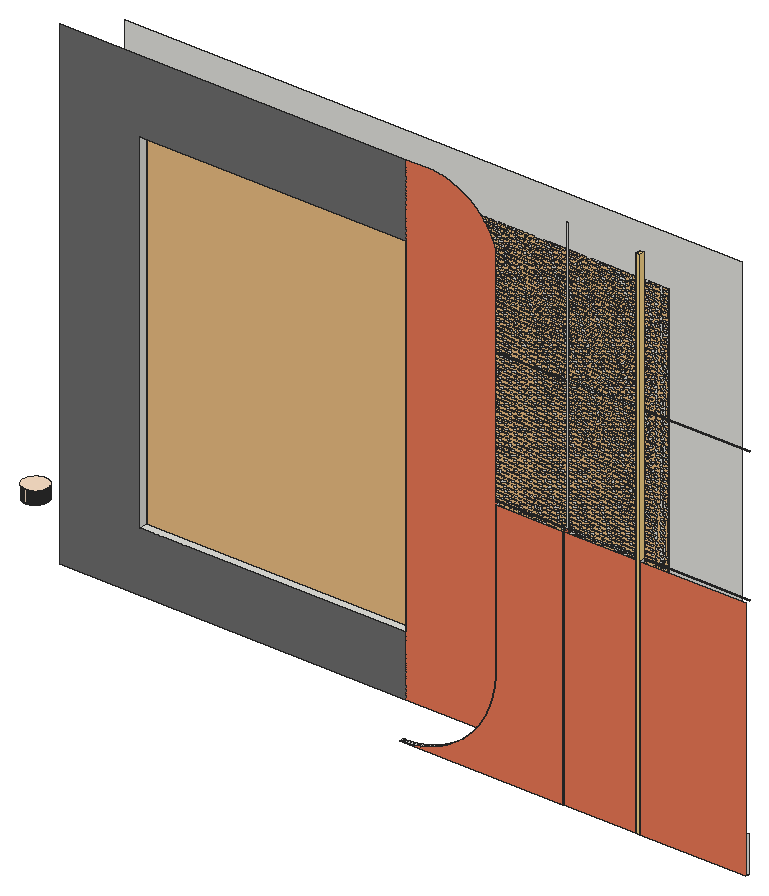
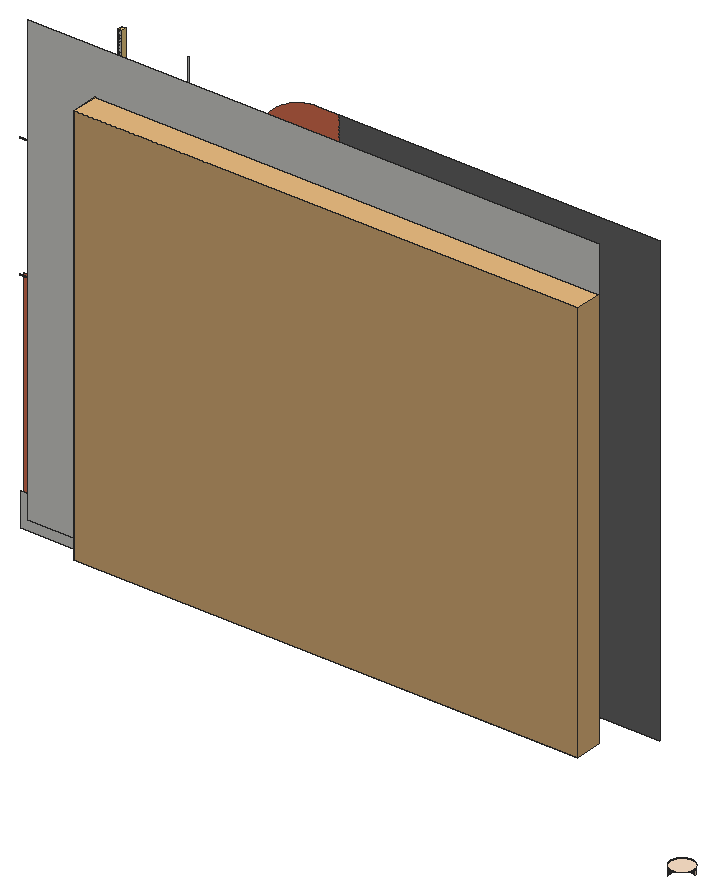
# SketchUp Ruby script. Lengths in inches.
U = 1.inch
M = Sketchup.active_model
def pt(a) = Geom::Point3d.new(a.map { |v| v * U })
def face(e, loops, mat)
  f = e.add_face(loops[0].map { |a| pt(a) })
  loops[1..].each { |l| e.add_face(l.map { |a| pt(a) }).erase! }
  f.material = f.back_material = mat if mat
  f
end
# faces: each face lists its corners as indices into pts; further lists are holes
def faces(e, pts, list, mat = nil) = list.each { |f| face(e, (f[0].is_a?(Array) ? f : [f]).map { |l| l.map { |i| pts[i] } }, mat) }
# xy, xz, yz: faces in a plane at the given z, y or x. An outline is a flat list of corners, or four numbers for a rectangle; further outlines are holes
def ring(l) = l.size == 4 ? [[l[0], l[1]], [l[2], l[1]], [l[2], l[3]], [l[0], l[3]]] : l.each_slice(2).to_a
def flat(e, list, mat, &to3) = list.each { |f| face(e, (f[0].is_a?(Array) ? f : [f]).map { |l| ring(l).map { |u, v| to3.(u, v) } }, mat) }
def xy(e, z, list, mat = nil) = flat(e, list, mat) { |x, y| [x, y, z] }
def xz(e, y, list, mat = nil) = flat(e, list, mat) { |x, z| [x, y, z] }
def yz(e, x, list, mat = nil) = flat(e, list, mat) { |y, z| [x, y, z] }
def lines(e, pts, list) = list.each { |a, b| e.add_line(pt(pts[a]), pt(pts[b])) }
# prism: a flat outline (further loops are holes) pulled along v
def prism(e, loops, v, mat = nil)
  f = face(e, loops, mat); d = Geom::Vector3d.new(v.map { |x| x * U })
  f.pushpull(f.normal.samedirection?(d) ? d.length : -d.length)
end
def box(e, o, s, mat = nil) = prism(e, [[o, [o[0] + s[0], o[1], o[2]], [o[0] + s[0], o[1] + s[1], o[2]], [o[0], o[1] + s[1], o[2]]]], [0, 0, s[2]], mat)
def at(x, y, z, deg = 0) = Geom::Transformation.translation(pt([x, y, z])) * Geom::Transformation.rotation(ORIGIN, Z_AXIS, deg.degrees)
def axes(o, x, y, z) = Geom::Transformation.new([*x, 0, *y, 0, *z, 0, *pt(o).to_a, 1])
def part(name) = M.definitions.add(name)
# library, detail: a bought-in or finely detailed component or shape, given as its bounding box
def library(name, o, s) = part(name).tap { |d| box(d.entities, o, s) }
def detail(e, o, s) = box(e.add_group.entities, o, s)
def put(e, d, t, mat = nil) = e.add_instance(d, t).tap { |i| i.material = mat if mat }
def group(e, t, mat = nil) = e.add_group.tap { |g| g.transformation = t; g.material = mat if mat }.entities
root = M.entities
M.materials.add("1122 AP 7994 PEACH ROSE").color = [254, 227, 201]
M.materials.add("Wall Light").color = [248, 213, 137]
M.materials.add("[Formica Beige]").color = [235, 120, 86]
M.materials.add("[Stone Flagstone Ashlar]").color = [109, 109, 109]
c1 = library("Component",[73.72,0,0],[62.99,4.72,84.625])
c2 = library("Component_63",[0,-41.05,1.35],[7.23,156.73,136.43])
xy(root,149.82,[[280.17,152,280.52,153],[280.17,152,320.75,153],[321,152,338.75,153],[339.75,152,366,153]])
xy(root,152.82,[[164.79,180.07,164.72,180.08,164.4,180.12,164.33,180.14,164.25,180.15,164.17,180.17,164.1,180.19,164.02,180.22,163.95,180.24,163.8,180.3,163.66,180.36,163.59,180.4,163.52,180.43,163.38,180.51,163.32,180.55,163.25,180.6,163.1875,180.64,163,180.79,162.94,180.84,162.83,180.95,162.78,181.01,162.72,181.0625,162.67,181.12,162.57,181.24,162.52,181.31,162.48,181.37,162.44,181.4375,162.39,181.5,162.31,181.64,162.28,181.71,162.24,181.78,162.18,181.92,162.15,182,162.1,182.14,162.07,182.22,162.05,182.29,162.03,182.37,162.02,182.45,162,182.52,161.96,182.84,161.96,182.91,161.95,182.99,161.95,183.15,161.96,183.23,161.96,183.31,161.97,183.38,162,183.62,162.02,183.69,162.03,183.77,162.05,183.85,162.07,183.92,162.1,184,162.125,184.07,162.15,184.15,162.24,184.36,162.28,184.43,162.31,184.5,162.39,184.64,162.44,184.7,162.48,184.77,162.52,184.83,162.57,184.9,162.72,185.08,162.94,185.3,163,185.35,163.1875,185.5,163.25,185.54,163.32,185.59,163.38,185.63,163.52,185.71,163.59,185.74,163.66,185.78,163.73,185.8125,163.8,185.84,163.95,185.9,164.02,185.92,164.1,185.95,164.17,185.97,164.33,186.01,164.4,186.02,164.48,186.03,164.56,186.05,164.64,186.05,164.72,186.0625,164.79,186.07,165.11,186.07,165.1875,186.0625,165.26,186.05,165.34,186.05,165.42,186.03,165.5,186.02,165.57,186.01,165.73,185.97,165.8,185.95,165.88,185.92,165.95,185.9,166.03,185.87,166.1,185.84,166.17,185.8125,166.24,185.78,166.3125,185.74,166.38,185.71,166.59,185.59,166.65,185.54,166.71,185.5,166.78,185.45,167.02,185.25,167.07,185.19,167.13,185.14,167.33,184.9,167.38,184.83,167.42,184.77,167.47,184.7,167.51,184.64,167.59,184.5,167.66,184.36,167.75,184.15,167.78,184.07,167.8,184,167.83,183.92,167.85,183.85,167.89,183.69,167.9,183.62,167.91,183.54,167.93,183.46,167.93,183.38,167.94,183.31,167.95,183.23,167.95,182.91,167.94,182.84,167.93,182.76,167.93,182.68,167.91,182.6,167.9,182.52,167.89,182.45,167.85,182.29,167.83,182.22,167.8,182.14,167.78,182.07,167.75,182,167.72,181.92,167.66,181.78,167.59,181.64,167.51,181.5,167.47,181.4375,167.42,181.37,167.38,181.31,167.33,181.24,167.23,181.12,167.18,181.0625,167.13,181.01,167.07,180.95,167.02,180.89,166.78,180.69,166.71,180.64,166.65,180.6,166.59,180.55,166.38,180.43,166.3125,180.4,166.24,180.36,166.03,180.27,165.95,180.24,165.88,180.22,165.8,180.19,165.73,180.17,165.65,180.15,165.57,180.14,165.5,180.12,165.26,180.09,165.1875,180.08,165.11,180.07]],"1122 AP 7994 PEACH ROSE")
xy(root,173.82,[[215,153,281,162]])
xz(root,152,[[280.17,149.82,320.75,149.82,320.75,210.57,304,210.57,304,173.17,303.99,172.85,303.97,172.52,303.96,172.2,303.93,171.875,303.91,171.55,303.88,171.23,303.76,170.27,303.71,169.95,303.66,169.625,303.6,169.31,303.54,168.99,303.47,168.67,303.4,168.36,303.33,168.04,303.25,167.73,303.17,167.41,302.9,166.48,302.8,166.17,302.69,165.86,302.47,165.26,302.36,164.95,302.24,164.65,302.11,164.35,301.98,164.06,301.85,163.76,301.71,163.47,301.57,163.17,301.43,162.88,301.28,162.6,301.13,162.31,300.97,162.03,300.8125,161.74,300.65,161.46,300.48,161.1875,300.31,160.91,300.13,160.64,299.96,160.37,299.77,160.1,299.59,159.84,299.4,159.57,299.2,159.3125,299.01,159.06,298.79,158.82,298.58,158.52,298.36,158.25,298.12,157.98,297.89,157.71,297.65,157.45,297.4,157.1875,297.15,156.93,296.9,156.68,296.64,156.43,296.39,156.1875,296.12,155.95,295.86,155.71,295.58,155.48,295.3125,155.25,295.03,155.02,294.75,154.8,294.47,154.59,294.18,154.375,293.89,154.17,293.6,153.96,293.3,153.77,293,153.57,292.7,153.38,292.4,153.2,291.78,152.84,291.47,152.67,291.15,152.5,290.51,152.18,289.87,151.88,289.21,151.6,288.55,151.34,288.21,151.22,287.875,151.1,287.54,150.99,287.2,150.88,286.85,150.78,286.51,150.68,286.17,150.59,285.82,150.5,285.47,150.42,285.125,150.34,284.78,150.27,284.43,150.2,284.07,150.14,283.37,150.04,283.01,149.99,282.66,149.95,282.31,149.92,281.59,149.86,281.24,149.84,280.52,149.82],[321,149.82,338.75,210.57],[339.75,149.82,366,210.57]],"[Formica Beige]")
xz(root,153,[[280.17,149.82,280.52,149.82,280.88,149.83,281,149.83,281,149.82],[281,149.82,281,149.83,281.24,149.84,281.59,149.86,282.31,149.92,282.66,149.95,283.01,149.99,283.37,150.04,284.07,150.14,284.43,150.2,284.78,150.27,285.125,150.34,285.47,150.42,285.82,150.5,286.17,150.59,286.51,150.68,286.85,150.78,287.2,150.88,287.54,150.99,287.875,151.1,288.21,151.22,288.55,151.34,289.21,151.6,289.87,151.88,290.51,152.18,291.15,152.5,291.47,152.67,291.78,152.84,292.4,153.2,292.7,153.38,293,153.57,293.3,153.77,293.6,153.96,293.89,154.17,294.18,154.375,294.47,154.59,294.75,154.8,295.03,155.02,295.3125,155.25,295.58,155.48,295.86,155.71,296.12,155.95,296.39,156.1875,296.64,156.43,296.9,156.68,297.15,156.93,297.4,157.1875,297.65,157.45,297.89,157.71,298.12,157.98,298.36,158.25,298.58,158.52,298.79,158.82,320.75,158.82,320.75,149.82],[321,149.82,338.75,158.82],[339.75,149.82,366,158.82]])
xz(root,153,[[281,158.82,298.79,158.82,299.01,159.06,299.2,159.3125,299.4,159.57,299.59,159.84,299.77,160.1,299.96,160.37,300.13,160.64,300.31,160.91,300.48,161.1875,300.65,161.46,300.8125,161.74,300.97,162.03,301.13,162.31,301.28,162.6,301.43,162.88,301.57,163.17,301.71,163.47,301.85,163.76,301.98,164.06,302.11,164.35,302.24,164.65,302.36,164.95,302.47,165.26,302.69,165.86,302.8,166.17,302.9,166.48,303.17,167.41,303.25,167.73,303.33,168.04,303.4,168.36,303.47,168.67,303.54,168.99,303.6,169.31,303.66,169.625,303.71,169.95,303.76,170.27,303.88,171.23,303.91,171.55,303.93,171.875,303.96,172.2,303.97,172.52,303.99,172.85,304,173.17,304,210.57,303,210.57,303,266.72,302.94,267,302.85,267.26,302.75,267.52,302.64,267.77,302.54,268.03,302.42,268.28,302.31,268.54,302.1875,268.79,302.07,269.03,301.9375,269.28,301.81,269.52,301.67,269.77,301.53,270.01,301.39,270.24,301.24,270.48,301.1,270.71,300.94,270.94,300.79,271.17,300.625,271.4,300.46,271.62,300.29,271.84,300.12,272.0625,299.95,272.28,299.41,272.91,299.22,273.11,299.03,273.3125,298.84,273.51,298.64,273.71,298.24,274.09,298.03,274.28,297.4,274.82,296.74,275.33,296.52,275.49,296.29,275.65,296.0625,275.8,295.83,275.96,295.6,276.1,295.36,276.25,294.88,276.53,294.64,276.66,294.39,276.79,294.15,276.92,293.65,277.16,293.39,277.27,293.14,277.39,292.88,277.49,292.625,277.6,292.37,277.69,292.11,277.79,291.85,277.88,291.58,277.97,291.32,278.05,291.05,278.13,290.78,278.2,290.52,278.27,290.25,278.34,289.71,278.46,289.43,278.51,289.16,278.56,288.89,278.6,288.61,278.65,288.34,278.68,288.0625,278.71,287.79,278.74,287.51,278.77,287.23,278.78,286.96,278.8,286.68,278.8125,286.4,278.82,281,278.82]],"[Formica Beige]")
xz(root,153,[[195,158.82,281,158.82,281,173.82,215,173.82,215,260.82,281,260.82,281,278.82,195,278.82]],"[Stone Flagstone Ashlar]")
xz(root,153.25,[[[320.75,158.82,321,158.82,321,210.57,338.75,210.57,338.75,158.82,339.75,158.82,339.75,210.57,366,210.57,366,210.82,339.75,210.82,339.75,243.57,366,243.57,366,243.82,339.75,243.82,339.75,278.82,338.75,278.82,338.75,243.82,321,243.82,321,278.82,320.75,278.82,320.75,243.82,303,243.82,303,243.57,320.75,243.57,320.75,210.82,303,210.82,303,210.57,320.75,210.57],[321,210.82,338.75,243.57]]])
xz(root,162,[[[204,158.82,357,278.82],[215,173.82,281,260.82]]])
xz(root,180.07,[[164.79,149.82,164.87,152.82],[164.87,149.82,164.95,152.82],[164.95,149.82,165.03,152.82],[165.03,149.82,165.11,152.82]],"1122 AP 7994 PEACH ROSE")
yz(root,167.93,[[182.68,149.82,182.76,152.82],[183.38,149.82,183.46,152.82]],"1122 AP 7994 PEACH ROSE")
yz(root,167.95,[[182.91,149.82,182.99,152.82],[182.99,149.82,183.07,152.82],[183.07,149.82,183.15,152.82],[183.15,149.82,183.23,152.82]],"1122 AP 7994 PEACH ROSE")
yz(root,215,[[153,173.82,162,260.82]])
yz(root,281,[[153,173.82,162,260.82]])
yz(root,304,[[152,173.17,153,173.5],[152,173.5,153,173.65],[152,173.65,153,173.82],[152,173.82,153,210.57]])
yz(root,320.75,[[152,149.82,153,158.82]])
yz(root,320.75,[[152,158.82,153.25,210.57]],"[Formica Beige]")
yz(root,321,[[152,149.82,152,210.57,153.25,210.57,153.25,158.82,153,158.82,153,149.82]],"[Formica Beige]")
yz(root,338.75,[[152,149.82,153,149.82,153,158.82,153.25,158.82,153.25,210.57,152,210.57]])
yz(root,339.75,[[152,149.82,152,210.57,153.25,210.57,153.25,158.82,153,158.82,153,149.82]])
p = [[280.88,153,149.83],[280.52,153,149.82],[280.52,152,149.82],[280.88,152,149.83],[281,153,149.83],[281.24,152,149.84],
  [281.24,153,149.84],[281.59,153,149.86],[281.59,152,149.86],[164.33,180.14,149.82],[164.25,180.15,149.82],[164.25,180.15,152.82],
  [164.33,180.14,152.82],[164.4,180.12,149.82],[164.4,180.12,152.82],[164.48,180.11,149.82],[164.48,180.11,152.82],[164.56,180.1,149.82],
  [164.56,180.1,152.82],[164.64,180.09,149.82],[164.64,180.09,152.82],[164.72,180.08,149.82],[164.72,180.08,152.82],[164.79,180.07,149.82],
  [164.79,180.07,152.82],[165.1875,180.08,149.82],[165.11,180.07,149.82],[165.11,180.07,152.82],[165.1875,180.08,152.82],[165.26,180.09,149.82],
  [165.26,180.09,152.82],[165.34,180.1,149.82],[165.34,180.1,152.82],[165.42,180.11,149.82],[165.42,180.11,152.82],[165.5,180.12,149.82],
  [165.5,180.12,152.82],[165.57,180.14,149.82],[165.57,180.14,152.82],[165.65,180.15,149.82],[165.65,180.15,152.82],[163.95,180.24,149.82],
  [163.875,180.27,149.82],[163.875,180.27,152.82],[163.95,180.24,152.82],[164.02,180.22,149.82],[164.02,180.22,152.82],[164.1,180.19,149.82],
  [164.1,180.19,152.82],[164.17,180.17,149.82],[164.17,180.17,152.82],[165.73,180.17,149.82],[165.73,180.17,152.82],[165.8,180.19,149.82],
  [165.8,180.19,152.82],[165.88,180.22,149.82],[165.88,180.22,152.82],[165.95,180.24,149.82],[165.95,180.24,152.82],[166.03,180.27,149.82],
  [166.03,180.27,152.82],[163.73,180.33,149.82],[163.66,180.36,149.82],[163.66,180.36,152.82],[163.73,180.33,152.82],[163.8,180.3,149.82],
  [163.8,180.3,152.82],[166.1,180.3,149.82],[166.1,180.3,152.82],[166.17,180.33,149.82],[166.17,180.33,152.82],[166.24,180.36,149.82],
  [166.24,180.36,152.82],[163.52,180.43,149.82],[163.45,180.47,149.82],[163.45,180.47,152.82],[163.52,180.43,152.82],[163.59,180.4,149.82],
  [163.59,180.4,152.82],[166.3125,180.4,149.82],[166.3125,180.4,152.82],[166.38,180.43,149.82],[166.38,180.43,152.82],[166.45,180.47,149.82],
  [166.45,180.47,152.82],[166.52,180.51,149.82],[166.52,180.51,152.82],[166.59,180.55,149.82],[166.59,180.55,152.82],[166.65,180.6,149.82],
  [166.65,180.6,152.82],[166.71,180.64,149.82],[166.71,180.64,152.82],[166.78,180.69,149.82],[166.78,180.69,152.82],[166.84,180.74,149.82],
  [166.84,180.74,152.82],[166.9,180.79,149.82],[166.9,180.79,152.82],[166.96,180.84,149.82],[166.96,180.84,152.82],[167.02,180.89,149.82],
  [167.02,180.89,152.82],[167.07,180.95,149.82],[167.07,180.95,152.82],[167.13,181.01,149.82],[167.13,181.01,152.82],[167.18,181.0625,149.82],
  [167.18,181.0625,152.82],[167.23,181.12,149.82],[167.23,181.12,152.82],[167.28,181.18,149.82],[167.28,181.18,152.82],[167.33,181.24,149.82],
  [167.33,181.24,152.82],[167.38,181.31,149.82],[167.38,181.31,152.82],[167.42,181.37,149.82],[167.42,181.37,152.82],[167.47,181.4375,149.82],
  [167.47,181.4375,152.82],[167.51,181.5,149.82],[167.51,181.5,152.82],[167.55,181.57,149.82],[167.55,181.57,152.82],[167.59,181.64,149.82],
  [167.59,181.64,152.82],[167.625,181.71,149.82],[167.625,181.71,152.82],[167.66,181.78,149.82],[167.66,181.78,152.82],[167.69,181.85,149.82],
  [167.69,181.85,152.82],[167.72,181.92,149.82],[167.72,181.92,152.82],[167.75,182,149.82],[167.75,182,152.82],[167.78,182.07,149.82],
  [167.78,182.07,152.82],[167.8,182.14,149.82],[167.8,182.14,152.82],[167.83,182.22,149.82],[167.83,182.22,152.82],[167.85,182.29,149.82],
  [167.85,182.29,152.82],[167.87,182.37,149.82],[167.87,182.37,152.82],[167.89,182.45,149.82],[167.89,182.45,152.82],[167.9,182.52,149.82],
  [167.9,182.52,152.82],[167.91,182.6,149.82],[167.91,182.6,152.82],[167.93,182.68,149.82],[167.93,182.68,152.82],[167.94,182.84,149.82],
  [167.93,182.76,149.82],[167.93,182.76,152.82],[167.94,182.84,152.82],[167.95,182.91,149.82],[167.95,182.91,152.82],[167.94,183.31,149.82],
  [167.95,183.23,149.82],[167.95,183.23,152.82],[167.94,183.31,152.82],[167.93,183.38,149.82],[167.93,183.38,152.82],[167.9,183.62,149.82],
  [167.91,183.54,149.82],[167.91,183.54,152.82],[167.9,183.62,152.82],[167.93,183.46,149.82],[167.93,183.46,152.82],[167.89,183.69,149.82],
  [167.89,183.69,152.82],[167.87,183.77,149.82],[167.87,183.77,152.82],[167.83,183.92,149.82],[167.85,183.85,149.82],[167.85,183.85,152.82],
  [167.83,183.92,152.82],[167.8,184,149.82],[167.8,184,152.82],[167.78,184.07,149.82],[167.78,184.07,152.82],[167.72,184.22,149.82],
  [167.75,184.15,149.82],[167.75,184.15,152.82],[167.72,184.22,152.82],[167.69,184.29,149.82],[167.69,184.29,152.82],[167.66,184.36,149.82],
  [167.66,184.36,152.82],[281.95,153,149.89],[281.95,152,149.89],[282.31,153,149.92],[282.31,152,149.92],[282.66,153,149.95],
  [282.66,152,149.95],[283.01,153,149.99],[283.01,152,149.99],[283.37,153,150.04],[283.37,152,150.04],[283.72,153,150.09],
  [283.72,152,150.09],[284.07,153,150.14],[284.07,152,150.14],[284.43,153,150.2],[284.43,152,150.2],[284.78,153,150.27],
  [284.78,152,150.27],[285.125,153,150.34],[285.125,152,150.34],[285.47,153,150.42],[285.47,152,150.42],[285.82,153,150.5],
  [285.82,152,150.5],[286.17,153,150.59],[286.17,152,150.59],[286.51,153,150.68],[286.51,152,150.68],[286.85,153,150.78],
  [286.85,152,150.78],[287.2,153,150.88],[287.2,152,150.88],[287.54,153,150.99],[287.54,152,150.99],[287.875,153,151.1],
  [287.875,152,151.1],[288.21,153,151.22],[288.21,152,151.22],[288.55,153,151.34],[288.55,152,151.34],[288.88,153,151.47],
  [288.88,152,151.47],[289.21,153,151.6],[289.21,152,151.6],[289.54,153,151.74],[289.54,152,151.74],[289.87,153,151.88],
  [289.87,152,151.88],[290.19,153,152.03],[290.19,152,152.03],[290.51,153,152.18],[290.51,152,152.18],[290.83,153,152.34],
  [290.83,152,152.34],[291.15,153,152.5],[291.15,152,152.5],[291.47,153,152.67],[291.47,152,152.67],[291.78,153,152.84],
  [291.78,152,152.84],[292.09,153,153.02],[292.09,152,153.02],[292.4,153,153.2],[292.4,152,153.2],[292.7,153,153.38],
  [292.7,152,153.38],[293,153,153.57],[293,152,153.57],[293.3,153,153.77],[293.3,152,153.77],[293.6,153,153.96],
  [293.6,152,153.96],[293.89,153,154.17],[293.89,152,154.17],[294.18,153,154.375],[294.18,152,154.375],[294.47,153,154.59],
  [294.47,152,154.59],[294.75,153,154.8],[294.75,152,154.8],[295.03,153,155.02],[295.03,152,155.02],[295.3125,153,155.25],
  [295.3125,152,155.25],[295.58,153,155.48],[295.58,152,155.48],[295.86,153,155.71],[295.86,152,155.71],[296.12,153,155.95],
  [296.12,152,155.95],[296.39,153,156.1875],[296.39,152,156.1875],[296.64,153,156.43],[296.64,152,156.43],[296.9,153,156.68],
  [296.9,152,156.68],[297.15,153,156.93],[297.15,152,156.93],[297.4,153,157.1875],[297.4,152,157.1875],[297.65,153,157.45],
  [297.65,152,157.45],[297.89,153,157.71],[297.89,152,157.71],[298.12,153,157.98],[298.12,152,157.98],[298.36,153,158.25],
  [298.36,152,158.25],[298.58,153,158.52],[298.58,152,158.52],[298.79,153,158.82],[298.79,152,158.82],[299.01,153,159.06],
  [299.01,152,159.06],[299.2,153,159.3125],[299.2,152,159.3125],[299.4,153,159.57],[299.4,152,159.57],[299.59,153,159.84],
  [299.59,152,159.84],[299.77,153,160.1],[299.77,152,160.1],[299.96,153,160.37],[299.96,152,160.37],[300.13,153,160.64],
  [300.13,152,160.64],[300.31,153,160.91],[300.31,152,160.91],[300.48,153,161.1875],[300.48,152,161.1875],[300.65,153,161.46],
  [300.65,152,161.46],[300.8125,153,161.74],[300.8125,152,161.74],[300.97,153,162.03],[300.97,152,162.03],[301.13,153,162.31],
  [301.13,152,162.31],[301.28,153,162.6],[301.28,152,162.6],[301.43,153,162.88],[301.43,152,162.88],[301.57,153,163.17],
  [301.57,152,163.17],[301.71,153,163.47],[301.71,152,163.47],[301.85,153,163.76],[301.85,152,163.76],[301.98,153,164.06],
  [301.98,152,164.06],[302.11,153,164.35],[302.11,152,164.35],[302.24,153,164.65],[302.24,152,164.65],[302.36,153,164.95],
  [302.36,152,164.95],[302.47,153,165.26],[302.47,152,165.26],[302.58,153,165.56],[302.58,152,165.56],[302.69,153,165.86],
  [302.69,152,165.86],[302.8,153,166.17],[302.8,152,166.17],[302.9,153,166.48],[302.9,152,166.48],[302.99,153,166.79],
  [302.99,152,166.79],[303.08,153,167.1],[303.08,152,167.1],[303.17,153,167.41],[303.17,152,167.41],[303.25,153,167.73],
  [303.25,152,167.73],[303.33,153,168.04],[303.33,152,168.04],[303.4,153,168.36],[303.4,152,168.36],[303.47,153,168.67],
  [303.47,152,168.67],[303.54,153,168.99],[303.54,152,168.99],[303.6,153,169.31],[303.6,152,169.31],[303.66,153,169.625],
  [303.66,152,169.625],[303.71,153,169.95],[303.71,152,169.95],[303.76,153,170.27],[303.76,152,170.27],[303.8,153,170.59],
  [303.8,152,170.59],[303.84,153,170.91],[303.84,152,170.91],[303.88,153,171.23],[303.88,152,171.23],[303.91,153,171.55],
  [303.91,152,171.55],[303.93,153,171.875],[303.93,152,171.875],[303.96,153,172.2],[303.96,152,172.2],[303.97,153,172.52],
  [303.97,152,172.52],[303.99,153,172.85],[303.99,152,172.85],[304,153,173.17],[304,152,173.17]]
faces(root,p,[[0,1,2,3],[4,0,3,5,6],[7,6,5,8],[193,7,8,194],[195,193,194,196],[197,195,196,198],[199,197,198,200],[201,199,200,202],
  [203,201,202,204],[205,203,204,206],[207,205,206,208],[209,207,208,210],[211,209,210,212],[213,211,212,214],[215,213,214,216],[217,215,216,218],
  [219,217,218,220],[221,219,220,222],[223,221,222,224],[225,223,224,226],[227,225,226,228],[229,227,228,230],[231,229,230,232],[233,231,232,234],
  [235,233,234,236],[237,235,236,238],[239,237,238,240],[241,239,240,242],[243,241,242,244],[245,243,244,246],[247,245,246,248],[249,247,248,250],
  [251,249,250,252],[253,251,252,254],[255,253,254,256],[257,255,256,258],[259,257,258,260],[261,259,260,262],[263,261,262,264],[265,263,264,266],
  [267,265,266,268],[269,267,268,270],[271,269,270,272],[273,271,272,274],[275,273,274,276],[277,275,276,278],[279,277,278,280],[281,279,280,282],
  [283,281,282,284],[285,283,284,286],[287,285,286,288],[289,287,288,290],[291,289,290,292],[293,291,292,294],[295,293,294,296],[297,295,296,298],
  [299,297,298,300],[301,299,300,302],[303,301,302,304],[305,303,304,306],[307,305,306,308],[309,307,308,310],[311,309,310,312],[313,311,312,314],
  [315,313,314,316],[317,315,316,318],[319,317,318,320],[321,319,320,322],[323,321,322,324],[325,323,324,326],[327,325,326,328],[329,327,328,330],
  [331,329,330,332],[333,331,332,334],[335,333,334,336],[337,335,336,338],[339,337,338,340],[341,339,340,342],[343,341,342,344],[345,343,344,346],
  [347,345,346,348],[349,347,348,350],[351,349,350,352],[353,351,352,354],[355,353,354,356],[357,355,356,358],[359,357,358,360],[361,359,360,362],
  [363,361,362,364],[365,363,364,366],[367,365,366,368],[369,367,368,370],[371,369,370,372],[373,371,372,374],[375,373,374,376],[377,375,376,378],
  [379,377,378,380],[381,379,380,382],[383,381,382,384],[385,383,384,386],[387,385,386,388],[389,387,388,390],[391,389,390,392],[393,391,392,394],
  [395,393,394,396],[397,395,396,398],[399,397,398,400]])
faces(root,p,[[9,10,11,12],[13,9,12,14],[15,13,14,16],[17,15,16,18],[19,17,18,20],[21,19,20,22],[23,21,22,24],[25,26,27,28],
  [29,25,28,30],[31,29,30,32],[33,31,32,34],[35,33,34,36],[37,35,36,38],[39,37,38,40],[41,42,43,44],[45,41,44,46],
  [47,45,46,48],[49,47,48,50],[10,49,50,11],[51,39,40,52],[53,51,52,54],[55,53,54,56],[57,55,56,58],[59,57,58,60],
  [61,62,63,64],[65,61,64,66],[42,65,66,43],[67,59,60,68],[69,67,68,70],[71,69,70,72],[73,74,75,76],[77,73,76,78],
  [62,77,78,63],[79,71,72,80],[81,79,80,82],[83,81,82,84],[85,83,84,86],[87,85,86,88],[89,87,88,90],[91,89,90,92],
  [93,91,92,94],[95,93,94,96],[97,95,96,98],[99,97,98,100],[101,99,100,102],[103,101,102,104],[105,103,104,106],[107,105,106,108],
  [109,107,108,110],[111,109,110,112],[113,111,112,114],[115,113,114,116],[117,115,116,118],[119,117,118,120],[121,119,120,122],[123,121,122,124],
  [125,123,124,126],[127,125,126,128],[129,127,128,130],[131,129,130,132],[133,131,132,134],[135,133,134,136],[137,135,136,138],[139,137,138,140],
  [141,139,140,142],[143,141,142,144],[145,143,144,146],[147,145,146,148],[149,147,148,150],[151,149,150,152],[153,151,152,154],[155,156,157,158],
  [159,155,158,160],[161,162,163,164],[165,161,164,166],[167,168,169,170],[168,171,172,169],[173,167,170,174],[175,173,174,176],[177,178,179,180],
  [178,175,176,179],[181,177,180,182],[183,181,182,184],[185,186,187,188],[186,183,184,187],[189,185,188,190],[191,189,190,192]],"1122 AP 7994 PEACH ROSE")
put(root,c1,axes([137.76,159.72,173.82],[1.04775,0,0],[0,-1,0],[0,0,1.02805]))
put(root,c2,axes([303.64,162,267.67],[0,1,0],[-0.86133,0,0],[0,0,-0.79]))
g1 = group(root,at(338.75,153.25,149.82),"Wall Light")
box(g1,[0,-1.25,0],[1,1.25,129])
